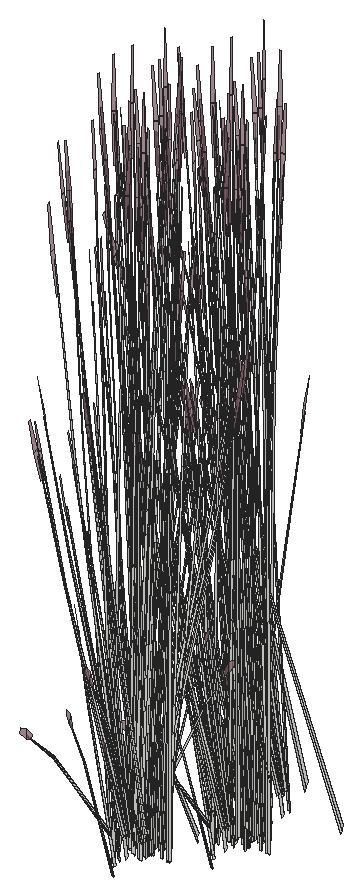
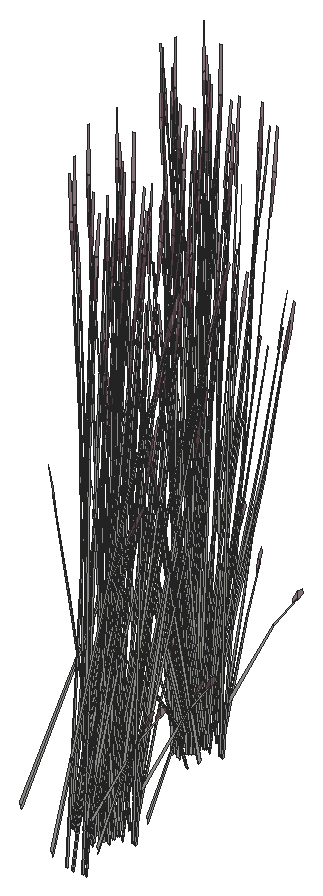
# SketchUp Ruby script. Lengths in inches.
U = 1.inch
M = Sketchup.active_model
def pt(a) = Geom::Point3d.new(a.map { |v| v * U })
def face(e, loops, mat)
  f = e.add_face(loops[0].map { |a| pt(a) })
  loops[1..].each { |l| e.add_face(l.map { |a| pt(a) }).erase! }
  f.material = f.back_material = mat if mat
  f
end
# faces: each face lists its corners as indices into pts; further lists are holes
def faces(e, pts, list, mat = nil) = list.each { |f| face(e, (f[0].is_a?(Array) ? f : [f]).map { |l| l.map { |i| pts[i] } }, mat) }
# xy, xz, yz: faces in a plane at the given z, y or x. An outline is a flat list of corners, or four numbers for a rectangle; further outlines are holes
def ring(l) = l.size == 4 ? [[l[0], l[1]], [l[2], l[1]], [l[2], l[3]], [l[0], l[3]]] : l.each_slice(2).to_a
def flat(e, list, mat, &to3) = list.each { |f| face(e, (f[0].is_a?(Array) ? f : [f]).map { |l| ring(l).map { |u, v| to3.(u, v) } }, mat) }
def xy(e, z, list, mat = nil) = flat(e, list, mat) { |x, y| [x, y, z] }
def xz(e, y, list, mat = nil) = flat(e, list, mat) { |x, z| [x, y, z] }
def yz(e, x, list, mat = nil) = flat(e, list, mat) { |y, z| [x, y, z] }
def lines(e, pts, list) = list.each { |a, b| e.add_line(pt(pts[a]), pt(pts[b])) }
# prism: a flat outline (further loops are holes) pulled along v
def prism(e, loops, v, mat = nil)
  f = face(e, loops, mat); d = Geom::Vector3d.new(v.map { |x| x * U })
  f.pushpull(f.normal.samedirection?(d) ? d.length : -d.length)
end
def box(e, o, s, mat = nil) = prism(e, [[o, [o[0] + s[0], o[1], o[2]], [o[0] + s[0], o[1] + s[1], o[2]], [o[0], o[1] + s[1], o[2]]]], [0, 0, s[2]], mat)
def at(x, y, z, deg = 0) = Geom::Transformation.translation(pt([x, y, z])) * Geom::Transformation.rotation(ORIGIN, Z_AXIS, deg.degrees)
def axes(o, x, y, z) = Geom::Transformation.new([*x, 0, *y, 0, *z, 0, *pt(o).to_a, 1])
def part(name) = M.definitions.add(name)
# library, detail: a bought-in or finely detailed component or shape, given as its bounding box
def library(name, o, s) = part(name).tap { |d| box(d.entities, o, s) }
def detail(e, o, s) = box(e.add_group.entities, o, s)
def put(e, d, t, mat = nil) = e.add_instance(d, t).tap { |i| i.material = mat if mat }
def group(e, t, mat = nil) = e.add_group.tap { |g| g.transformation = t; g.material = mat if mat }.entities
root = M.entities
M.materials.add("LightPink_Translucent").color = [144, 107, 117]
M.materials["LightPink_Translucent"].alpha = 0.75
c1 = part("blade")
p = [[2.15,0.21,22],[0,0.17,0],[0.09,0.45,0],[2.18,0.31,22],[2.29,0.31,22],[0.38,0.45,0],
  [2.48,0.24,33],[2.49,0.24,33],[2.48,0.22,33]]
faces(c1.entities,p,[[0,1,2,3],[4,5,2,3],[6,3,4,7],[8,0,3,6]])
c2 = part("seeds")
p = [[0.3,-0.1,1.38],[-0.01,-0.03,1.59],[-0.01,-0.03,0.03],[0.14,-0.07,-0.07],[0.29,-0.03,3],[0.15,0.01,3.11]]
faces(c2.entities,p,[[0,1,2,3],[1,0,4,5]],"LightPink_Translucent")
c3 = part("blade with seeds")
put(c3.entities,c1,at(0,0,0))
put(c3.entities,c2,axes([2.4,0.25,30.99],[1.5799,-0.05474,1.17369],[-0.12525,1.92788,0.29478],[-0.07173,-0.02425,1.56792]))
put(root,c3,axes([313.96,14.3,49.36],[-0.07723,-0.05479,1.54581],[-0.51538,0.03473,-0.24447],[-0.08225,-0.13104,0.12397]))
put(root,c3,axes([314.5,15.23,49.6],[-0.24099,-0.31773,-0.62776],[0.49607,-0.17707,0.07576],[-0.05635,-0.15352,0.88802]))
put(root,c3,axes([314.08,14.53,46.52],[-0.08469,0.01408,1.55816],[-0.46834,-0.15847,-0.23804],[0.00786,-0.13218,0.26541]))
put(root,c3,axes([314.54,14.96,49.2],[0.15222,-0.30049,-0.31292],[0.44409,0.08764,0.40398],[-0.04072,-0.12098,0.77298]))
put(root,c3,axes([316.16,14.7,49.36],[-0.05128,0.02985,1.56736],[-0.5024,-0.1007,-0.1481],[-0.01819,-0.13025,0.27737]))
put(root,c3,axes([314.32,15.17,49.33],[-0.49634,-0.09796,-0.45151],[0.17013,-0.33585,-0.34973],[-0.04551,-0.13522,0.86392]))
put(root,c3,axes([314.625,14.33,47.64],[0.06477,0.22786,1.01491],[-0.35932,-0.1262,0.74569],[0.03867,-0.11667,0.22354]))
put(root,c3,axes([314.6,15.03,49.38],[0.49753,0.10215,0.42415],[-0.17013,0.33585,0.34973],[-0.0299,-0.13207,0.87768]))
put(root,c3,axes([314.74,15.15,49.64],[-0.49409,0.18193,-0.10745],[-0.24281,-0.32289,-0.59638],[-0.06519,-0.13607,0.90619]))
put(root,c3,axes([315.77,15.56,49.64],[-0.55492,-0.01936,-0.10745],[0.01517,-0.36657,-0.59638],[0.03855,-0.14118,0.90619]))
put(root,c3,axes([314.73,15,49.375],[0.37205,-0.1328,0.05682],[0.18211,0.24217,0.44729],[-0.03593,-0.10675,0.68204]))
put(root,c3,axes([313.38,16.42,47.05],[-0.20736,-0.4007,-0.61707],[0.59731,-0.14431,-0.16195],[-0.02292,-0.13569,1.36206]))
put(root,c3,axes([314.59,15.28,49.66],[-0.15222,0.30049,0.31292],[-0.44409,-0.08764,-0.40398],[-0.04072,-0.12098,0.77298]))
put(root,c3,axes([313.3,15.27,47.29],[-0.31568,-0.39156,0],[0.52815,-0.21836,-0.456],[0.12029,-0.04973,1.44655]))
put(root,c3,axes([314,14.8,47.08],[-0.34892,0.22417,-0.0344],[-0.3197,-0.24551,-0.15595],[-0.02251,-0.06957,0.51438]))
put(root,c3,axes([312.16,16.37,46.98],[0,-0.39075,-0.43871],[0.56491,0,0],[0,-0.089,1.3917]))
put(root,c3,axes([313.7,16.53,47.15],[0.24498,-0.3521,-0.39531],[0.50902,0.16945,0.19025],[0,-0.08116,1.26923]))
put(root,c3,axes([312.4,16.375,46.99],[0.35245,-0.2438,-0.27372],[0.35245,0.2438,0.27372],[0,-0.07853,1.22797]))
put(root,c3,axes([313.64,16.82,47.55],[-0.56863,-0.18645,-0.25709],[0.2738,-0.39352,-0.44182],[-0.01787,-0.09662,1.41118]))
put(root,c3,axes([314,16.7,47.35],[0.56891,0.18939,0.21263],[-0.2738,0.39352,0.44182],[0,-0.09071,1.41855]))
put(root,c3,axes([313.78,17.23,47.35],[0.13383,-0.46302,-0.20702],[0.63453,0.08071,0.45303],[-0.11087,-0.06394,1.38231]))
put(root,c3,axes([313.82,16.4375,47.6],[-0.54829,0.02412,0.39531],[-0.04958,-0.40041,-0.19025],[0.09816,-0.04058,1.26923]))
put(root,c3,axes([312.4,16.73,47.39],[0,0.39075,0.43871],[-0.56491,0,0],[0,-0.089,1.3917]))
put(root,c3,axes([313.8,16.58,47.28],[0.21952,0.43694,0.40429],[-0.62724,0.15194,0.15865],[0.00767,-0.08029,1.40366]))
put(root,c3,axes([313.6875,16.93,47.6],[-0.24498,0.3521,0.39531],[-0.50902,-0.16945,-0.19025],[0,-0.08116,1.26923]))
put(root,c3,axes([314.59,16.62,47.14],[0,-0.45213,0],[0.63136,0,0],[0,0,1.58567]))
put(root,c3,axes([314.29,16.33,47.28],[-0.41865,0.35461,0.40429],[-0.49737,-0.31303,0.15865],[0.10093,-0.03539,1.40366]))
put(root,c3,axes([314.75,16.97,47.23],[-0.46965,-0.33633,-0.05417],[0.46994,-0.33653,0],[-0.0164,-0.01174,1.55135]))
put(root,c3,axes([313.5625,15.75,47.38],[-0.14586,0.38834,0.15589],[-0.53375,-0.1099,0.31002],[0.0922,-0.00189,1.41735]))
put(root,c3,axes([313.85,17.01,47.28],[0.63817,0.08233,0.40429],[-0.12987,0.46497,0.15865],[-0.09326,-0.0449,1.40366]))
put(root,c3,axes([313.51,17.75,47.38],[0.54257,-0.10371,0.15589],[0.13397,0.38597,0.31002],[-0.04839,-0.05624,1.41735]))
put(root,c3,axes([315.18,15.77,47.38],[-0.54257,0.10371,0.15589],[-0.13397,-0.38597,0.31002],[0.04839,0.05624,1.41735]))
put(root,c3,axes([314.84,16.51,47.3],[-0.63817,-0.08233,0.43472],[0.12987,-0.46497,0.17059],[0.09326,0.0449,1.50931]))
put(root,c3,axes([314.33,17.66,47.14],[-0.16474,-0.33688,0],[0.47043,-0.11798,0],[0,0,1.36402]))
put(root,c3,axes([314.01,17.34,47.51],[-0.09741,0.34873,0.12794],[-0.4759,-0.06053,-0.36534],[-0.08661,-0.03581,1.11991]))
put(root,c3,axes([315.125,17.77,47.38],[0.14586,-0.38834,0.15589],[0.53375,0.1099,0.31002],[-0.0922,0.00189,1.41735]))
put(root,c3,axes([315.01,16.89,47.15],[0.35245,0.2524,0],[-0.35245,0.2524,0],[0,0,1.49564]))
put(root,c3,axes([315.96,16.78,47.38],[-0.39671,-0.28463,0.15589],[0.39978,-0.27607,0.31002],[-0.04381,0.05813,1.41735]))
put(root,c3,axes([314.21,17.82,47.14],[-0.50902,-0.17543,0],[0.24498,-0.36452,0],[0,0,1.43768]))
put(root,c3,axes([315,16.6,47.6],[0.24498,-0.3521,0.39531],[0.50902,0.16945,-0.19025],[0,0.08116,1.26923]))
put(root,c3,axes([314.91,16.8,47.22],[0,0.45191,-0.04981],[-0.63136,0,0],[0,0.0142,1.58489]))
put(root,c3,axes([314.87,17.09,47.6],[0.54829,-0.02412,0.39531],[0.04958,0.40041,-0.19025],[-0.09816,0.04058,1.26923]))
put(root,c3,axes([314.79,17.82,47.14],[0.50902,0.17543,0],[-0.24498,0.36452,0],[0,0,1.54589]))
put(root,c3,axes([314.99,18.21,47.13],[-0.31175,-0.39292,-0.04544],[0.52815,-0.21836,0.456],[-0.13015,0.03741,1.44584]))
put(root,c3,axes([314.88,17.26,47.51],[0.37303,0.23477,0.12794],[-0.31115,0.26487,-0.36534],[-0.08661,0.03581,1.11991]))
put(root,c3,axes([315.28,17.98,47.39],[0.47255,-0.19538,0.43871],[0.28245,0.35034,0],[-0.10763,0.0445,1.3917]))
put(root,c3,axes([314.6,17.67,47.22],[0.21952,0.44891,-0.05313],[-0.62724,0.1573,0],[0.00767,0.01568,1.52132]))
put(root,c3,axes([314.85,18.16,46.99],[-0.47106,-0.09668,-0.27372],[0.11861,-0.34048,0.27372],[-0.09497,0.03926,1.22797]))
put(root,c3,axes([316.42,17.09,47.14],[-0.63105,-0.00312,-0.04397],[0,-0.43672,0.44129],[-0.01983,0.09942,1.3992]))
put(root,c3,axes([316.29,17.15,46.99],[-0.35245,0.2438,-0.27372],[-0.35245,-0.2438,0.27372],[0,0.07853,1.22797]))
put(root,c3,axes([314.77,17.17,47.55],[0.05884,0.44587,-0.25709],[-0.6128,0.02696,-0.44182],[-0.10791,0.05939,1.41118]))
put(root,c3,axes([314.99,17,47.15],[-0.24498,0.3521,-0.39531],[-0.50902,-0.16945,0.19025],[0,0.08116,1.26923]))
put(root,c3,axes([315,18.01,47.26],[0.63212,0.12701,0.27176],[-0.15814,0.45398,-0.32244],[-0.10462,0.05682,1.45692]))
put(root,c3,axes([314.96,18.31,46.98],[-0.47255,0.19538,-0.43871],[-0.28245,-0.35034,0],[-0.10763,0.0445,1.3917]))
put(root,c3,axes([312.83,17.84,49.66],[0.34164,-0.20573,0.31292],[0.3234,0.23491,-0.40398],[-0.04921,0.11936,0.77298]))
put(root,c3,axes([315.39,18.25,47.29],[0.31568,0.39156,0],[-0.52815,0.21836,-0.456],[-0.12029,0.04973,1.44655]))
put(root,c3,axes([315.12,16.7,47.71],[-0.01379,-0.36791,1.24828],[0.62424,0.09537,0.52853],[-0.14764,0.20132,1.17828]))
put(root,c3,axes([313.79,18.18,49.66],[0.15222,-0.30049,0.31292],[0.44409,0.08764,-0.40398],[0.04072,0.12098,0.77298]))
put(root,c3,axes([314.38,19.25,50.18],[0.34892,-0.22417,-0.05733],[0.3197,0.24551,-0.25992],[0.02251,0.06957,0.85731]))
put(root,c3,axes([313.65,18.45,49.375],[-0.37205,0.1328,0.05682],[-0.18211,-0.24217,0.44729],[0.03593,0.10675,0.68204]))
put(root,c3,axes([312.61,17.89,49.96],[0.55492,0.01936,-0.11927],[-0.01517,0.36657,-0.66198],[-0.03855,0.14118,1.00587]))
put(root,c3,axes([313.64,18.3,49.64],[0.49409,-0.18193,-0.10745],[0.24281,0.32289,-0.59638],[0.06519,0.13607,0.90619]))
put(root,c3,axes([313.78,18.42,49.67],[-0.49753,-0.10215,0.47081],[0.17013,-0.33585,0.3882],[0.0299,0.13207,0.97422]))
put(root,c3,axes([313.73,18.375,46.52],[0.08172,-0.02126,1.55816],[0.49154,0.11703,-0.23804],[0.01437,0.1319,0.26541]))
put(root,c3,axes([314.5,23.26,46.17],[-0.07723,-0.05479,1.54581],[-0.51538,0.03473,-0.24447],[-0.08225,-0.13104,0.12397]))
put(root,c3,axes([312.99,18.03,49.62],[0.36145,0.26255,-0.50118],[-0.38183,0.22994,-0.3882],[-0.055,0.1334,0.95895]))
put(root,c3,axes([315.04,24.18,46.4],[-0.24099,-0.31773,-0.62776],[0.49607,-0.17707,0.07576],[-0.05635,-0.15352,0.88802]))
put(root,c3,axes([312.6,18.43,47.69],[0.45869,-0.0692,0.0575],[0.10545,0.27878,-0.76259],[-0.02908,0.14112,0.68355]))
put(root,c3,axes([314.0625,18.29,49.33],[0.49634,0.09796,-0.45151],[-0.17013,0.33585,-0.34973],[0.04551,0.13522,0.86392]))
put(root,c3,axes([314.63,23.48,43.32],[-0.08469,0.01408,1.55816],[-0.46834,-0.15847,-0.23804],[0.00786,-0.13218,0.26541]))
put(root,c3,axes([313.84,18.49,49.2],[-0.15222,0.30049,-0.31292],[-0.44409,-0.08764,0.40398],[0.04072,0.12098,0.77298]))
put(root,c3,axes([315.09,23.91,46],[0.15222,-0.30049,-0.31292],[0.44409,0.08764,0.40398],[-0.04072,-0.12098,0.77298]))
put(root,c3,axes([313.4,17.66,48.62],[-0.01236,-0.14998,1.51428],[0.53562,0.09949,0.12244],[-0.03313,0.21373,0.64734]))
put(root,c3,axes([314.86,24.12,46.14],[-0.49634,-0.09796,-0.45151],[0.17013,-0.33585,-0.34973],[-0.04551,-0.13522,0.86392]))
put(root,c3,axes([313.88,18.22,49.6],[0.24099,0.31773,-0.62776],[-0.49607,0.17707,0.07576],[0.05635,0.15352,0.88802]))
put(root,c3,axes([313.52,19.03,49.36],[0.064,0.06292,1.54581],[0.51651,0.02472,-0.24447],[0.05194,0.13877,0.12397]))
put(root,c3,axes([313.875,23.91,46.5],[0.56246,-0.10044,0.47505],[0.09762,0.39398,0.3917],[-0.13228,-0.11611,0.983]))
put(root,c3,axes([315.15,23.98,46.18],[0.49753,0.10215,0.42415],[-0.17013,0.33585,0.34973],[-0.0299,-0.13207,0.87768]))
put(root,c3,axes([315.29,24.1,46.45],[-0.49409,0.18193,-0.10745],[-0.24281,-0.32289,-0.59638],[-0.06519,-0.13607,0.90619]))
put(root,c3,axes([313.32,23.55,44.44],[0.26338,0.136,1.01491],[-0.38358,0.08175,0.74569],[-0.08207,-0.10452,0.22354]))
put(root,c3,axes([315.28,23.95,46.18],[0.37205,-0.1328,0.05682],[0.18211,0.24217,0.44729],[-0.03593,-0.10675,0.68204]))
put(root,c3,axes([312.69,18.42,48.17],[0.01109,-0.20172,1.3638],[0.49896,0.10655,0.18846],[-0.04323,0.21498,0.64398]))
put(root,c3,axes([314,23.99,46.18],[0.22948,-0.24822,0.05682],[0.32679,0.14452,0.44729],[-0.10565,-0.07958,0.68204]))
put(root,c3,axes([313.93,25.375,43.85],[-0.20736,-0.4007,-0.61707],[0.59731,-0.14431,-0.16195],[-0.02292,-0.13569,1.36206]))
put(root,c3,axes([315.14,24.23,46.46],[-0.15222,0.30049,0.31292],[-0.44409,-0.08764,-0.40398],[-0.04072,-0.12098,0.77298]))
put(root,c3,axes([313.85,24.22,44.1],[-0.31568,-0.39156,0],[0.52815,-0.21836,-0.456],[0.12029,-0.04973,1.44655]))
put(root,c3,axes([314.54,23.75,43.88],[-0.34892,0.22417,-0.0344],[-0.3197,-0.24551,-0.15595],[-0.02251,-0.06957,0.51438]))
put(root,c3,axes([314.99,26.41,44.9375],[0.43633,0.15757,1.33654],[-0.42745,0.33945,0.52853],[-0.19146,-0.20119,1.12046]))
put(root,c3,axes([312.71,25.32,43.78],[0,-0.39075,-0.43871],[0.56491,0,0],[0,-0.089,1.3917]))
put(root,c3,axes([314.25,25.48,43.95],[0.24498,-0.3521,-0.39531],[0.50902,0.16945,0.19025],[0,-0.08116,1.26923]))
put(root,c3,axes([312.95,25.33,43.79],[0.35245,-0.2438,-0.27372],[0.35245,0.2438,0.27372],[0,-0.07853,1.22797]))
put(root,c3,axes([314.18,25.77,44.36],[-0.56863,-0.18645,-0.25709],[0.2738,-0.39352,-0.44182],[-0.01787,-0.09662,1.41118]))
put(root,c3,axes([314.55,25.65,44.15],[0.56891,0.18939,0.21263],[-0.2738,0.39352,0.44182],[0,-0.09071,1.41855]))
put(root,c3,axes([314.33,26.18,44.16],[0.13383,-0.46302,-0.20702],[0.63453,0.08071,0.45303],[-0.11087,-0.06394,1.38231]))
put(root,c3,axes([314.37,25.39,44.4],[-0.54829,0.02412,0.39531],[-0.04958,-0.40041,-0.19025],[0.09816,-0.04058,1.26923]))
put(root,c3,axes([312.95,25.68,44.19],[0,0.39075,0.43871],[-0.56491,0,0],[0,-0.089,1.3917]))
put(root,c3,axes([314.28,26,43.95],[-0.30332,-0.32798,-0.39531],[0.45944,-0.23096,0.19025],[-0.09816,-0.04058,1.26923]))
put(root,c3,axes([314.35,25.53,44.09],[0.21952,0.43694,0.40429],[-0.62724,0.15194,0.15865],[0.00767,-0.08029,1.40366]))
put(root,c3,axes([314.24,25.88,44.4],[-0.24498,0.3521,0.39531],[-0.50902,-0.16945,-0.19025],[0,-0.08116,1.26923]))
put(root,c3,axes([315.14,25.57,43.95],[0,-0.45213,0],[0.63136,0,0],[0,0,1.58567]))
put(root,c3,axes([315.29,25.92,44.03],[-0.46965,-0.33633,-0.05417],[0.46994,-0.33653,0],[-0.0164,-0.01174,1.55135]))
put(root,c3,axes([314.11,24.7,44.1875],[-0.14586,0.38834,0.15589],[-0.53375,-0.1099,0.31002],[0.0922,-0.00189,1.41735]))
put(root,c3,axes([314.4,25.96,44.09],[0.63817,0.08233,0.40429],[-0.12987,0.46497,0.15865],[-0.09326,-0.0449,1.40366]))
put(root,c3,axes([314.06,26.7,44.1875],[0.54257,-0.10371,0.15589],[0.13397,0.38597,0.31002],[-0.04839,-0.05624,1.41735]))
put(root,c3,axes([314.875,26.61,43.95],[-0.16474,-0.33688,0],[0.47043,-0.11798,0],[0,0,1.36402]))
put(root,c3,axes([314.56,26.29,44.3125],[-0.09741,0.34873,0.12794],[-0.4759,-0.06053,-0.36534],[-0.08661,-0.03581,1.11991]))
put(root,c3,axes([315.67,26.72,44.1875],[0.14586,-0.38834,0.15589],[0.53375,0.1099,0.31002],[-0.0922,0.00189,1.41735]))
put(root,c3,axes([314.49,28.76,46.17],[-0.07723,-0.05479,1.54581],[-0.51538,0.03473,-0.24447],[-0.08225,-0.13104,0.12397]))
put(root,c3,axes([316.51,25.73,44.1875],[-0.39671,-0.28463,0.15589],[0.39978,-0.27607,0.31002],[-0.04381,0.05813,1.41735]))
put(root,c3,axes([315.03,29.68,46.4],[-0.24099,-0.31773,-0.62776],[0.49607,-0.17707,0.07576],[-0.05635,-0.15352,0.88802]))
put(root,c3,axes([314.76,26.77,43.94],[-0.50902,-0.17543,0],[0.24498,-0.36452,0],[0,0,1.43768]))
put(root,c3,axes([315.18,26.3,44.18],[-0.49304,-0.31451,-0.2226],[0.41487,-0.35316,0.48713],[-0.13277,0.03679,1.48635]))
put(root,c3,axes([313.88,26.9,44.19],[0.47255,0.19538,0.43871],[-0.28245,0.35034,0],[-0.10763,-0.0445,1.3917]))
put(root,c3,axes([314.62,28.98,43.32],[-0.08469,0.01408,1.55816],[-0.46834,-0.15847,-0.23804],[0.00786,-0.13218,0.26541]))
put(root,c3,axes([315.45,25.75,44.03],[0,0.45191,-0.04981],[-0.63136,0,0],[0,0.0142,1.58489]))
put(root,c3,axes([315.08,29.41,46],[0.15222,-0.30049,-0.31292],[0.44409,0.08764,0.40398],[-0.04072,-0.12098,0.77298]))
put(root,c3,axes([315.42,26.04,44.4],[0.54829,-0.02412,0.39531],[0.04958,0.40041,-0.19025],[-0.09816,0.04058,1.26923]))
put(root,c3,axes([314.93,26.23,43.95],[-0.54829,0.02412,-0.39531],[-0.04958,-0.40041,0.19025],[-0.09816,0.04058,1.26923]))
put(root,c3,axes([314.85,29.62,46.14],[-0.49634,-0.09796,-0.45151],[0.17013,-0.33585,-0.34973],[-0.04551,-0.13522,0.86392]))
put(root,c3,axes([315.54,27.16,43.9375],[-0.31175,-0.39292,-0.04544],[0.52815,-0.21836,0.456],[-0.13015,0.03741,1.44584]))
put(root,c3,axes([313.86,29.41,46.5],[0.56246,-0.10044,0.47505],[0.09762,0.39398,0.3917],[-0.13228,-0.11611,0.983]))
put(root,c3,axes([315.43,26.21,44.3125],[0.37303,0.23477,0.12794],[-0.31115,0.26487,-0.36534],[-0.08661,0.03581,1.11991]))
put(root,c3,axes([315.13,29.48,46.18],[0.49753,0.10215,0.42415],[-0.17013,0.33585,0.34973],[-0.0299,-0.13207,0.87768]))
put(root,c3,axes([315.28,29.6,46.45],[-0.49409,0.18193,-0.10745],[-0.24281,-0.32289,-0.59638],[-0.06519,-0.13607,0.90619]))
put(root,c3,axes([313.3125,29.05,44.44],[0.26338,0.136,1.01491],[-0.38358,0.08175,0.74569],[-0.08207,-0.10452,0.22354]))
put(root,c3,axes([315.26,29.46,46.18],[0.37205,-0.1328,0.05682],[0.18211,0.24217,0.44729],[-0.03593,-0.10675,0.68204]))
put(root,c3,axes([315.82,26.93,44.19],[0.47255,-0.19538,0.43871],[0.28245,0.35034,0],[-0.10763,0.0445,1.3917]))
put(root,c3,axes([315.15,26.625,44.02],[0.21952,0.44891,-0.05313],[-0.62724,0.1573,0],[0.00767,0.01568,1.52132]))
put(root,c3,axes([315.39,27.11,43.79],[-0.47106,-0.09668,-0.27372],[0.11861,-0.34048,0.27372],[-0.09497,0.03926,1.22797]))
put(root,c3,axes([313.99,29.49,46.18],[0.22948,-0.24822,0.05682],[0.32679,0.14452,0.44729],[-0.10565,-0.07958,0.68204]))
put(root,c3,axes([316.96,26.04,43.94],[-0.63105,-0.00312,-0.04397],[0,-0.43672,0.44129],[-0.01983,0.09942,1.3992]))
put(root,c3,axes([313.92,30.875,43.85],[-0.20736,-0.4007,-0.61707],[0.59731,-0.14431,-0.16195],[-0.02292,-0.13569,1.36206]))
put(root,c3,axes([315.3125,26.125,44.36],[0.05884,0.44587,-0.25709],[-0.6128,0.02696,-0.44182],[-0.10791,0.05939,1.41118]))
put(root,c3,axes([315.54,25.95,43.95],[-0.24498,0.3521,-0.39531],[-0.50902,-0.16945,0.19025],[0,0.08116,1.26923]))
put(root,c3,axes([315.125,29.73,46.46],[-0.15222,0.30049,0.31292],[-0.44409,-0.08764,-0.40398],[-0.04072,-0.12098,0.77298]))
put(root,c3,axes([320.37,28.5625,45.43],[0.20943,-0.00885,1.51428],[-0.13893,0.38357,0.12244],[-0.29846,-0.02372,0.64734]))
put(root,c3,axes([313.84,29.72,44.1],[-0.31568,-0.39156,0],[0.52815,-0.21836,-0.456],[0.12029,-0.04973,1.44655]))
put(root,c3,axes([315.55,26.96,44.06],[0.63212,0.12701,0.27176],[-0.15814,0.45398,-0.32244],[-0.10462,0.05682,1.45692]))
put(root,c3,axes([314.53,29.25,43.88],[-0.34892,0.22417,-0.0344],[-0.3197,-0.24551,-0.15595],[-0.02251,-0.06957,0.51438]))
put(root,c3,axes([315.51,27.26,43.78],[-0.47255,0.19538,-0.43871],[-0.28245,-0.35034,0],[-0.10763,0.0445,1.3917]))
put(root,c3,axes([314.98,31.91,44.9375],[0.43633,0.15757,1.33654],[-0.42745,0.33945,0.52853],[-0.19146,-0.20119,1.12046]))
put(root,c3,axes([312.7,30.82,43.78],[0,-0.39075,-0.43871],[0.56491,0,0],[0,-0.089,1.3917]))
put(root,c3,axes([313.375,26.79,46.46],[0.34164,-0.20573,0.31292],[0.3234,0.23491,-0.40398],[-0.04921,0.11936,0.77298]))
put(root,c3,axes([315.93,27.2,44.1],[0.31568,0.39156,0],[-0.52815,0.21836,-0.456],[-0.12029,0.04973,1.44655]))
put(root,c3,axes([315.67,25.65,44.51],[-0.01379,-0.36791,1.24828],[0.62424,0.09537,0.52853],[-0.14764,0.20132,1.17828]))
put(root,c3,axes([314.33,27.125,46.46],[0.15222,-0.30049,0.31292],[0.44409,0.08764,-0.40398],[0.04072,0.12098,0.77298]))
put(root,c3,axes([314.23,30.98,43.95],[0.24498,-0.3521,-0.39531],[0.50902,0.16945,0.19025],[0,-0.08116,1.26923]))
put(root,c3,axes([312.9375,30.83,43.79],[0.35245,-0.2438,-0.27372],[0.35245,0.2438,0.27372],[0,-0.07853,1.22797]))
